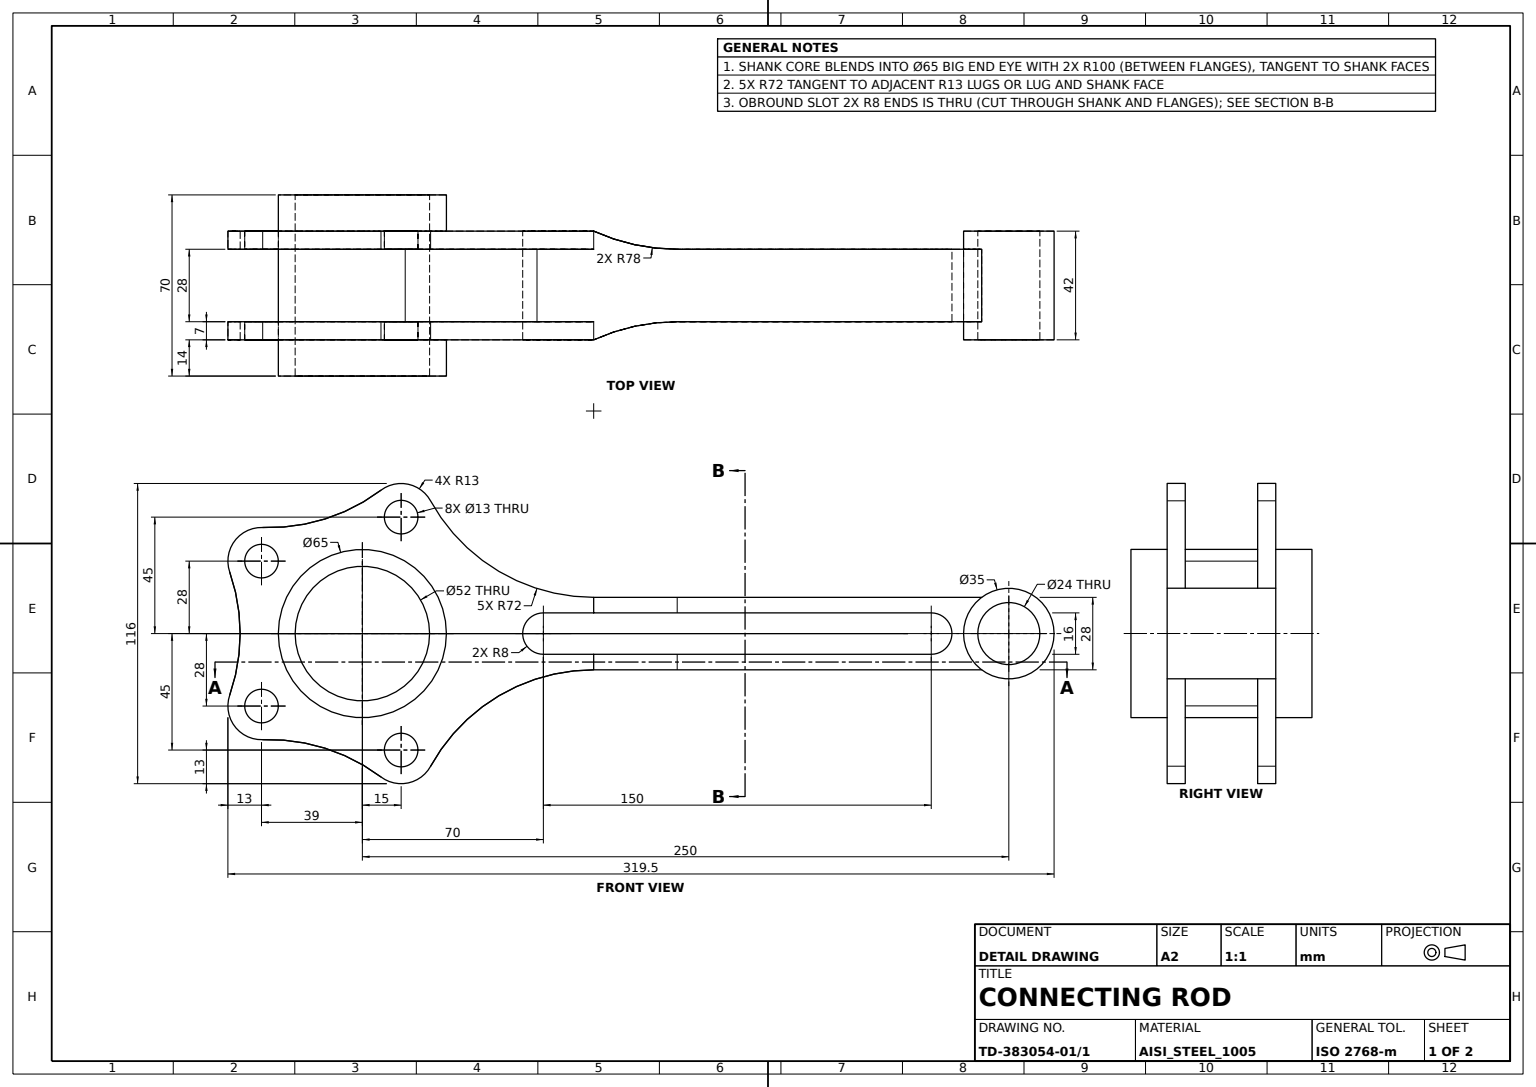
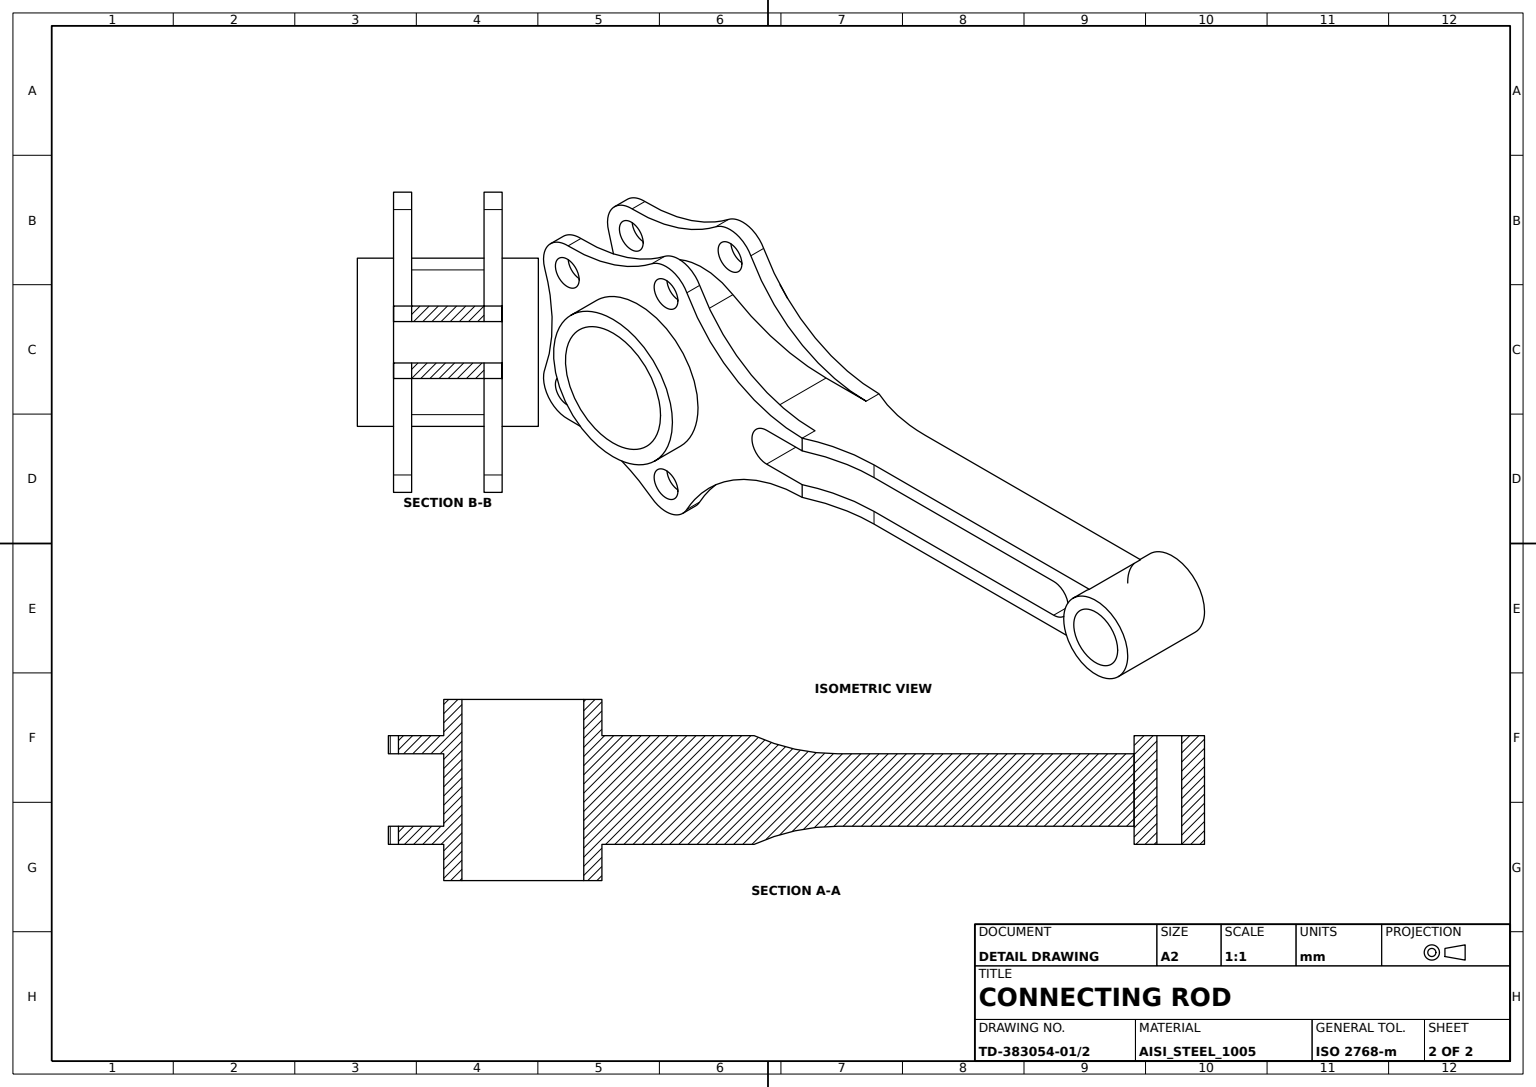
solid
v1 (26,-35,0)
e1 v1 v1 CIRCLE(AX(P(0,-35,0),D(0,1,0),D(1,0,0)),26)
v2 (26,35,0)
e2 v2 v2 CIRCLE(AX(P(0,35,0),D(0,1,0),D(1,0,0)),26)
face CYL(AX(P(0,-35,0),D(0,1,0),D(0,0,1)),26) rev [-e1] [e2]
v3 (121.753552,-14,8)
v4 (220,-14,8)
e3 v3 v4 LINE
v5 (220,-14,-8)
e4 v4 v5 CIRCLE(AX(P(220,-14,0),D(0,-1,0),D(0,0,-1)),8) rev
v6 (121.753552,-14,-8)
e5 v5 v6 LINE
v7 (121.753552,-14,-14)
e6 v6 v7 LINE
v8 (239.5,-14,-14)
e7 v8 v7 LINE
v9 (239.5,-14,14)
e8 v9 v8 CIRCLE(AX(P(250,-14,0),D(0,-1,0),D(1,0,0)),17.5)
v10 (121.753552,-14,14)
e9 v10 v9 LINE
e10 v10 v3 LINE
face PLANE(AX(P(250,-14,0),D(0,-1,0),D(0,0,-1))) [e3 e4 e5 e6 -e7 -e8 -e9 e10]
v11 (7.189691,21,-55.392261)
v12 (7.189691,14,-55.392261)
e11 v11 v12 LINE
v13 (-38.551485,14,-40.992261)
e12 v12 v13 CIRCLE(AX(P(-36.067402,14,-112.949396),D(0,-1,0),D(1,0,0)),72)
v14 (-38.551485,21,-40.992261)
e13 v14 v13 LINE
e14 v11 v14 CIRCLE(AX(P(-36.067402,21,-112.949396),D(0,-1,0),D(1,0,0)),72)
face CYL(AX(P(-36.067402,21,-112.949396),D(0,-1,0),D(0,0,-1)),72) rev [e11 e12 -e13 -e14]
v15 (21.5,-21,45)
e15 v15 v15 CIRCLE(AX(P(15,-21,45),D(0,1,0),D(1,0,0)),6.5)
v16 (21.5,-14,45)
e16 v16 v16 CIRCLE(AX(P(15,-14,45),D(0,1,0),D(1,0,0)),6.5)
face CYL(AX(P(15,-21,45),D(0,1,0),D(0,0,1)),6.5) rev [-e15] [e16]
v17 (32.5,-35,0)
e17 v17 v17 CIRCLE(AX(P(0,-35,0),D(0,1,0),D(1,0,0)),32.5)
face PLANE(AX(P(0,-35,0),D(0,1,0),D(0,0,1))) rev [e1] [-e17]
v18 (32.5,35,0)
e18 v18 v18 CIRCLE(AX(P(0,35,0),D(0,1,0),D(1,0,0)),32.5)
face PLANE(AX(P(0,35,0),D(0,1,0),D(0,0,1))) [-e2] [e18]
v19 (26.387701,21,-51.270588)
v20 (26.387701,14,-51.270588)
e19 v19 v20 LINE
e20 v20 v12 CIRCLE(AX(P(15,14,-45),D(0,1,0),D(1,0,0)),13)
e21 v19 v11 CIRCLE(AX(P(15,21,-45),D(0,1,0),D(1,0,0)),13)
face CYL(AX(P(15,21,-45),D(0,-1,0),D(0,0,-1)),13) [e19 e20 -e11 -e21]
v21 (-32.5,14,28)
e22 v21 v21 CIRCLE(AX(P(-39,14,28),D(0,1,0),D(1,0,0)),6.5)
v22 (21.5,14,45)
e23 v22 v22 CIRCLE(AX(P(15,14,45),D(0,1,0),D(1,0,0)),6.5)
v23 (89.458042,14,-14)
e24 v23 v20 CIRCLE(AX(P(89.458042,14,-86),D(0,-1,0),D(1,0,0)),72)
v24 (67.529623,14,-14)
e25 v23 v24 LINE
v25 (16.56387,14,-27.962264)
e26 v24 v25 CIRCLE(AX(P(67.529623,14,-114),D(0,-1,0),D(0,0,-1)),100)
v26 (16.56387,14,27.962264)
e27 v25 v26 CIRCLE(AX(P(0,14,0),D(0,-1,0),D(0,0,-1)),32.5) rev
v27 (67.529623,14,14)
e28 v26 v27 CIRCLE(AX(P(67.529623,14,114),D(0,-1,0),D(0,0,-1)),100)
v28 (89.458042,14,14)
e29 v27 v28 LINE
v29 (26.387701,14,51.270588)
e30 v29 v28 CIRCLE(AX(P(89.458042,14,86),D(0,-1,0),D(1,0,0)),72)
v30 (7.189691,14,55.392261)
e31 v30 v29 CIRCLE(AX(P(15,14,45),D(0,1,0),D(1,0,0)),13)
v31 (-38.551485,14,40.992261)
e32 v31 v30 CIRCLE(AX(P(-36.067402,14,112.949396),D(0,-1,0),D(1,0,0)),72)
v32 (-51.274423,14,23.717647)
e33 v32 v31 CIRCLE(AX(P(-39,14,28),D(0,1,0),D(1,0,0)),13)
v33 (-51.274423,14,-23.717647)
e34 v33 v32 CIRCLE(AX(P(-119.255841,14,0),D(0,-1,0),D(1,0,0)),72)
e35 v13 v33 CIRCLE(AX(P(-39,14,-28),D(0,1,0),D(1,0,0)),13)
v34 (21.5,14,-45)
e36 v34 v34 CIRCLE(AX(P(15,14,-45),D(0,-1,0),D(1,0,0)),6.5)
v35 (-32.5,14,-28)
e37 v35 v35 CIRCLE(AX(P(-39,14,-28),D(0,-1,0),D(1,0,0)),6.5)
face PLANE(AX(P(89.458042,14,86),D(0,-1,0),D(0,0,-1))) [e22] [e23] [-e20 -e24 e25 e26 e27 e28 e29 -e30 -e31 -e32 -e33 -e34 -e35 -e12] [-e36] [-e37]
v36 (-51.274423,-14,-23.717647)
v37 (-51.274423,-14,23.717647)
e38 v36 v37 CIRCLE(AX(P(-119.255841,-14,0),D(0,-1,0),D(1,0,0)),72)
v38 (-51.274423,-21,-23.717647)
e39 v38 v36 LINE
v39 (-51.274423,-21,23.717647)
e40 v38 v39 CIRCLE(AX(P(-119.255841,-21,0),D(0,-1,0),D(1,0,0)),72)
e41 v39 v37 LINE
face CYL(AX(P(-119.255841,-21,0),D(0,1,0),D(0,0,1)),72) rev [-e38 -e39 e40 e41]
v40 (-38.551485,21,40.992261)
e42 v40 v31 LINE
v41 (-51.274423,21,23.717647)
e43 v41 v40 CIRCLE(AX(P(-39,21,28),D(0,1,0),D(1,0,0)),13)
e44 v41 v32 LINE
face CYL(AX(P(-39,21,28),D(0,-1,0),D(0,0,-1)),13) [-e42 -e43 e44 e33]
v42 (21.5,21,-45)
e45 v42 v42 CIRCLE(AX(P(15,21,-45),D(0,-1,0),D(1,0,0)),6.5)
face CYL(AX(P(15,21,-45),D(0,-1,0),D(0,0,-1)),6.5) rev [e36] [-e45]
v43 (21.5,21,45)
e46 v43 v43 CIRCLE(AX(P(15,21,45),D(0,1,0),D(1,0,0)),6.5)
face CYL(AX(P(15,21,45),D(0,-1,0),D(0,0,-1)),6.5) rev [-e23] [e46]
v44 (16.56387,-14,27.962264)
e47 v44 v26 LINE
v45 (16.56387,-14,-27.962264)
e48 v25 v45 LINE
e49 v45 v44 CIRCLE(AX(P(0,-14,0),D(0,-1,0),D(0,0,-1)),32.5) rev
face CYL(AX(P(0,-35,0),D(0,1,0),D(0,0,1)),32.5) [e47 -e27 e48 e49]
v46 (89.458042,21,-14)
e50 v23 v46 LINE
v47 (121.753552,14,-14)
e51 v46 v47 CIRCLE(AX(P(121.753552,92,-14),D(0,0,-1),D(-1,0,0)),78) rev
v48 (239.5,14,-14)
e52 v48 v47 LINE
e53 v8 v48 LINE
v49 (89.458042,-21,-14)
e54 v7 v49 CIRCLE(AX(P(121.753552,-92,-14),D(0,0,-1),D(-1,0,0)),78) rev
v50 (89.458042,-14,-14)
e55 v50 v49 LINE
v51 (67.529623,-14,-14)
e56 v50 v51 LINE
e57 v51 v24 LINE
face PLANE(AX(P(239.5,-14,-14),D(0,0,-1),D(-1,0,0))) [-e25 e50 e51 -e52 -e53 e7 e54 -e55 e56 e57]
v52 (89.458042,-21,-8)
e58 v52 v49 LINE
e59 v52 v6 CIRCLE(AX(P(121.753552,-92,-8),D(0,0,1),D(1,0,0)),78) rev
face CYL(AX(P(121.753552,-92,14),D(0,0,-1),D(-1,0,0)),78) rev [e58 -e54 -e6 -e59]
v53 (7.189691,21,55.392261)
v54 (26.387701,21,51.270588)
e60 v53 v54 CIRCLE(AX(P(15,21,45),D(0,1,0),D(1,0,0)),13)
e61 v53 v30 LINE
e62 v54 v29 LINE
face CYL(AX(P(15,21,45),D(0,-1,0),D(0,0,-1)),13) [-e60 e61 e31 -e62]
v55 (-51.274423,21,-23.717647)
e63 v55 v33 LINE
e64 v14 v55 CIRCLE(AX(P(-39,21,-28),D(0,1,0),D(1,0,0)),13)
face CYL(AX(P(-39,21,-28),D(0,-1,0),D(0,0,-1)),13) [e13 e35 -e63 -e64]
v56 (89.458042,21,14)
e65 v28 v56 LINE
e66 v54 v56 CIRCLE(AX(P(89.458042,21,86),D(0,-1,0),D(1,0,0)),72)
face CYL(AX(P(89.458042,21,86),D(0,-1,0),D(0,0,-1)),72) rev [e30 e65 -e66 e62]
v57 (0,21,-32.5)
e67 v57 v57 CIRCLE(AX(P(0,21,0),D(0,-1,0),D(0,0,-1)),32.5) rev
face CYL(AX(P(0,-35,0),D(0,1,0),D(0,0,1)),32.5) [-e18] [e67]
v58 (7.189691,-14,55.392261)
v59 (26.387701,-14,51.270588)
e68 v58 v59 CIRCLE(AX(P(15,-14,45),D(0,1,0),D(1,0,0)),13)
v60 (7.189691,-21,55.392261)
e69 v60 v58 LINE
v61 (26.387701,-21,51.270588)
e70 v60 v61 CIRCLE(AX(P(15,-21,45),D(0,1,0),D(1,0,0)),13)
e71 v61 v59 LINE
face CYL(AX(P(15,-21,45),D(0,1,0),D(0,0,1)),13) [-e68 -e69 e70 e71]
v62 (7.189691,-14,-55.392261)
v63 (-38.551485,-14,-40.992261)
e72 v62 v63 CIRCLE(AX(P(-36.067402,-14,-112.949396),D(0,-1,0),D(1,0,0)),72)
e73 v63 v36 CIRCLE(AX(P(-39,-14,-28),D(0,1,0),D(1,0,0)),13)
v64 (-38.551485,-14,40.992261)
e74 v37 v64 CIRCLE(AX(P(-39,-14,28),D(0,1,0),D(1,0,0)),13)
e75 v64 v58 CIRCLE(AX(P(-36.067402,-14,112.949396),D(0,-1,0),D(1,0,0)),72)
v65 (89.458042,-14,14)
e76 v59 v65 CIRCLE(AX(P(89.458042,-14,86),D(0,-1,0),D(1,0,0)),72)
v66 (67.529623,-14,14)
e77 v66 v65 LINE
e78 v66 v44 CIRCLE(AX(P(67.529623,-14,114),D(0,-1,0),D(0,0,-1)),100) rev
e79 v45 v51 CIRCLE(AX(P(67.529623,-14,-114),D(0,-1,0),D(0,0,-1)),100) rev
v67 (26.387701,-14,-51.270588)
e80 v50 v67 CIRCLE(AX(P(89.458042,-14,-86),D(0,-1,0),D(1,0,0)),72)
e81 v67 v62 CIRCLE(AX(P(15,-14,-45),D(0,1,0),D(1,0,0)),13)
v68 (-32.5,-14,-28)
e82 v68 v68 CIRCLE(AX(P(-39,-14,-28),D(0,-1,0),D(1,0,0)),6.5)
v69 (21.5,-14,-45)
e83 v69 v69 CIRCLE(AX(P(15,-14,-45),D(0,-1,0),D(1,0,0)),6.5)
v70 (-32.5,-14,28)
e84 v70 v70 CIRCLE(AX(P(-39,-14,28),D(0,1,0),D(1,0,0)),6.5)
face PLANE(AX(P(89.458042,-14,86),D(0,-1,0),D(0,0,-1))) rev [e72 e73 e38 e74 e75 e68 e76 -e77 e78 -e49 e79 -e56 e80 e81] [e82] [e83] [-e16] [-e84]
v71 (220,14,8)
v72 (220,14,-8)
e85 v71 v72 CIRCLE(AX(P(220,14,0),D(0,-1,0),D(0,0,-1)),8) rev
v73 (121.753552,14,8)
e86 v73 v71 LINE
v74 (121.753552,14,14)
e87 v73 v74 LINE
v75 (239.5,14,14)
e88 v74 v75 LINE
e89 v75 v48 CIRCLE(AX(P(250,14,0),D(0,-1,0),D(1,0,0)),17.5)
v76 (121.753552,14,-8)
e90 v47 v76 LINE
e91 v72 v76 LINE
face PLANE(AX(P(250,14,0),D(0,-1,0),D(0,0,-1))) rev [-e85 -e86 e87 e88 e89 e52 e90 -e91]
v77 (-32.5,21,-28)
e92 v77 v77 CIRCLE(AX(P(-39,21,-28),D(0,-1,0),D(1,0,0)),6.5)
face CYL(AX(P(-39,21,-28),D(0,-1,0),D(0,0,-1)),6.5) rev [e37] [-e92]
e93 v27 v66 LINE
v78 (89.458042,-21,14)
e94 v65 v78 LINE
e95 v78 v10 CIRCLE(AX(P(121.753552,-92,14),D(0,0,1),D(1,0,0)),78) rev
e96 v9 v75 LINE
e97 v74 v56 CIRCLE(AX(P(121.753552,92,14),D(0,0,1),D(1,0,0)),78) rev
face PLANE(AX(P(29.330019,-14,14),D(0,0,1),D(1,0,0))) [e93 e77 e94 e95 e9 e96 -e88 e97 -e65 -e29]
face CYL(AX(P(67.529623,-35,-114),D(0,1,0),D(0,0,1)),100) rev [-e26 -e57 -e79 -e48]
v79 (0,-21,-32.5)
e98 v79 v79 CIRCLE(AX(P(0,-21,0),D(0,-1,0),D(0,0,-1)),32.5) rev
face CYL(AX(P(0,-35,0),D(0,1,0),D(0,0,1)),32.5) [-e98] [e17]
v80 (-38.551485,-21,-40.992261)
e99 v80 v63 LINE
v81 (7.189691,-21,-55.392261)
e100 v81 v62 LINE
e101 v81 v80 CIRCLE(AX(P(-36.067402,-21,-112.949396),D(0,-1,0),D(1,0,0)),72)
face CYL(AX(P(-36.067402,-21,-112.949396),D(0,1,0),D(0,0,1)),72) rev [e99 -e72 -e100 e101]
e102 v46 v19 CIRCLE(AX(P(89.458042,21,-86),D(0,-1,0),D(1,0,0)),72)
face CYL(AX(P(89.458042,21,-86),D(0,-1,0),D(0,0,-1)),72) rev [-e102 -e50 e24 -e19]
v82 (-38.551485,-21,40.992261)
e103 v82 v64 LINE
e104 v82 v60 CIRCLE(AX(P(-36.067402,-21,112.949396),D(0,-1,0),D(1,0,0)),72)
face CYL(AX(P(-36.067402,-21,112.949396),D(0,1,0),D(0,0,1)),72) rev [e69 -e75 -e103 e104]
e105 v55 v41 CIRCLE(AX(P(-119.255841,21,0),D(0,-1,0),D(1,0,0)),72)
face CYL(AX(P(-119.255841,21,0),D(0,-1,0),D(0,0,-1)),72) rev [e34 -e44 -e105 e63]
face CYL(AX(P(67.529623,-35,114),D(0,1,0),D(0,0,1)),100) rev [-e78 -e93 -e28 -e47]
v83 (89.458042,21,-8)
e106 v83 v46 LINE
e107 v76 v83 CIRCLE(AX(P(121.753552,92,-8),D(0,0,1),D(1,0,0)),78) rev
face CYL(AX(P(121.753552,92,14),D(0,0,1),D(1,0,0)),78) rev [-e51 -e106 -e107 -e90]
v84 (89.458042,-21,8)
e108 v3 v84 CIRCLE(AX(P(121.753552,-92,8),D(0,0,-1),D(-1,0,0)),78) rev
e109 v78 v84 LINE
face CYL(AX(P(121.753552,-92,14),D(0,0,-1),D(-1,0,0)),78) rev [-e108 -e10 -e95 e109]
v85 (89.458042,21,8)
v86 (70,21,8)
e110 v85 v86 LINE
e111 v85 v73 CIRCLE(AX(P(121.753552,92,8),D(0,0,-1),D(-1,0,0)),78) rev
e112 v71 v4 LINE
v87 (70,-21,8)
e113 v84 v87 LINE
e114 v86 v87 LINE
face PLANE(AX(P(220,-21,8),D(0,0,-1),D(-1,0,0))) [-e110 e111 e86 e112 -e3 e108 e113 -e114]
e115 v61 v78 CIRCLE(AX(P(89.458042,-21,86),D(0,-1,0),D(1,0,0)),72)
face CYL(AX(P(89.458042,-21,86),D(0,1,0),D(0,0,1)),72) rev [-e71 e115 -e94 -e76]
face CYL(AX(P(250,-14,0),D(0,1,0),D(0,0,1)),17.5) rev [e8 e53 -e89 -e96]
v88 (21.5,-21,-45)
e116 v88 v88 CIRCLE(AX(P(15,-21,-45),D(0,-1,0),D(1,0,0)),6.5)
face CYL(AX(P(15,-21,-45),D(0,1,0),D(0,0,1)),6.5) rev [-e83] [e116]
e117 v40 v53 CIRCLE(AX(P(-36.067402,21,112.949396),D(0,-1,0),D(1,0,0)),72)
face CYL(AX(P(-36.067402,21,112.949396),D(0,-1,0),D(0,0,-1)),72) rev [-e61 -e117 e42 e32]
v89 (26.387701,-21,-51.270588)
e118 v49 v89 CIRCLE(AX(P(89.458042,-21,-86),D(0,-1,0),D(1,0,0)),72)
e119 v89 v67 LINE
face CYL(AX(P(89.458042,-21,-86),D(0,1,0),D(0,0,1)),72) rev [-e80 e55 e118 e119]
e120 v39 v82 CIRCLE(AX(P(-39,-21,28),D(0,1,0),D(1,0,0)),13)
face CYL(AX(P(-39,-21,28),D(0,1,0),D(0,0,1)),13) [-e74 -e41 e120 e103]
e121 v89 v81 CIRCLE(AX(P(15,-21,-45),D(0,1,0),D(1,0,0)),13)
face CYL(AX(P(15,-21,-45),D(0,1,0),D(0,0,1)),13) [e121 e100 -e81 -e119]
v90 (-32.5,21,28)
e122 v90 v90 CIRCLE(AX(P(-39,21,28),D(0,1,0),D(1,0,0)),6.5)
e123 v56 v85 LINE
v91 (70,21,-8)
e124 v86 v91 CIRCLE(AX(P(70,21,0),D(0,-1,0),D(1,0,0)),8)
e125 v91 v83 LINE
face PLANE(AX(P(89.458042,21,86),D(0,-1,0),D(0,0,-1))) rev [e92] [-e67] [-e46] [-e122] [e106 e102 e21 e14 e64 e105 e43 e117 e60 e66 e123 e110 e124 e125] [e45]
e126 v72 v5 LINE
v92 (70,-21,-8)
e127 v91 v92 LINE
e128 v92 v52 LINE
face PLANE(AX(P(70,-21,-8),D(0,0,1),D(1,0,0))) [-e5 -e126 e91 e107 -e125 e127 e128 e59]
v93 (-32.5,-21,-28)
e129 v93 v93 CIRCLE(AX(P(-39,-21,-28),D(0,-1,0),D(1,0,0)),6.5)
face CYL(AX(P(-39,-21,-28),D(0,1,0),D(0,0,1)),6.5) rev [e129] [-e82]
face CYL(AX(P(220,-21,0),D(0,1,0),D(0,0,1)),8) rev [e126 -e4 -e112 e85]
e130 v87 v92 CIRCLE(AX(P(70,-21,0),D(0,-1,0),D(1,0,0)),8)
face CYL(AX(P(70,-21,0),D(0,1,0),D(0,0,1)),8) rev [-e127 -e124 e114 e130]
face CYL(AX(P(121.753552,92,14),D(0,0,1),D(1,0,0)),78) rev [-e111 -e123 -e97 -e87]
e131 v80 v38 CIRCLE(AX(P(-39,-21,-28),D(0,1,0),D(1,0,0)),13)
face CYL(AX(P(-39,-21,-28),D(0,1,0),D(0,0,1)),13) [e39 -e73 -e99 e131]
face CYL(AX(P(-39,21,28),D(0,-1,0),D(0,0,-1)),6.5) rev [-e22] [e122]
v94 (-32.5,-21,28)
e132 v94 v94 CIRCLE(AX(P(-39,-21,28),D(0,1,0),D(1,0,0)),6.5)
face PLANE(AX(P(89.458042,-21,86),D(0,-1,0),D(0,0,-1))) [e15] [e132] [-e131 -e101 -e121 -e118 -e58 -e128 -e130 -e113 -e109 -e115 -e70 -e104 -e120 -e40] [-e116] [e98] [-e129]
face CYL(AX(P(-39,-21,28),D(0,1,0),D(0,0,1)),6.5) rev [-e132] [e84]
solid
v95 (262,-21,0)
e133 v95 v95 CIRCLE(AX(P(250,-21,0),D(0,-1,0),D(1,0,0)),12)
v96 (267.5,-21,0)
e134 v96 v96 CIRCLE(AX(P(250,-21,0),D(0,-1,0),D(1,0,0)),17.5)
face PLANE(AX(P(250,-21,0),D(0,-1,0),D(0,0,-1))) [-e133] [e134]
v97 (267.5,21,0)
e135 v97 v97 CIRCLE(AX(P(250,21,0),D(0,-1,0),D(1,0,0)),17.5)
v98 (262,21,0)
e136 v98 v98 CIRCLE(AX(P(250,21,0),D(0,-1,0),D(1,0,0)),12)
face PLANE(AX(P(250,21,0),D(0,-1,0),D(0,0,-1))) rev [-e135] [e136]
face CYL(AX(P(250,-21,0),D(0,1,0),D(0,0,1)),12) rev [e133] [-e136]
face CYL(AX(P(250,-21,0),D(0,1,0),D(0,0,1)),17.5) [e135] [-e134]
